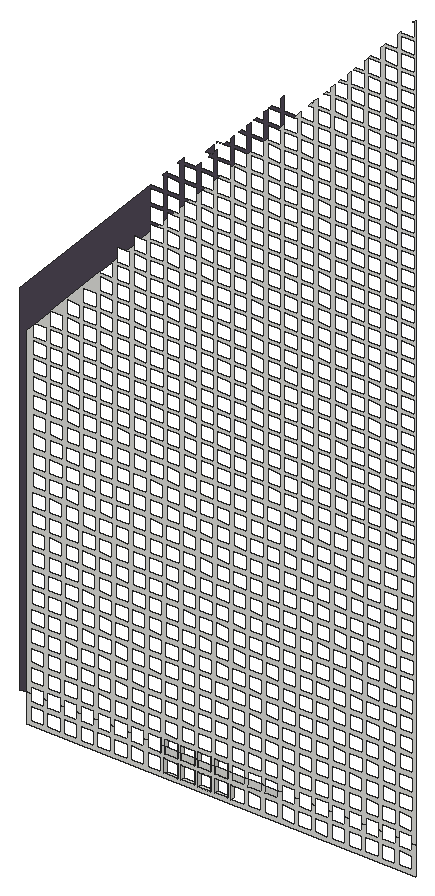
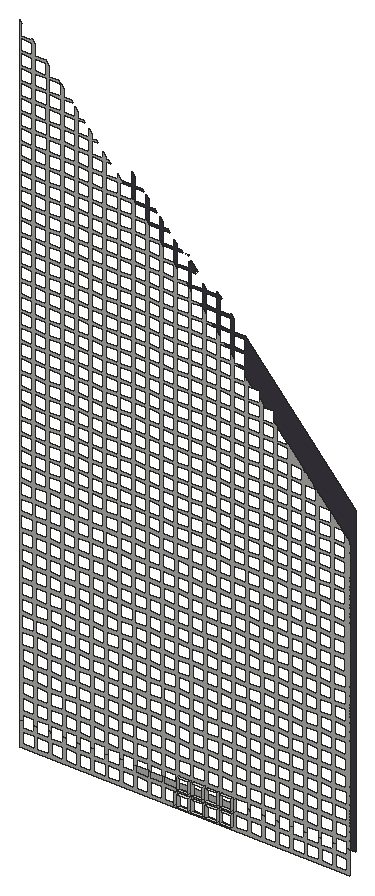
# SketchUp Ruby script. Lengths in inches.
U = 1.inch
M = Sketchup.active_model
def pt(a) = Geom::Point3d.new(a.map { |v| v * U })
def face(e, loops, mat)
  f = e.add_face(loops[0].map { |a| pt(a) })
  loops[1..].each { |l| e.add_face(l.map { |a| pt(a) }).erase! }
  f.material = f.back_material = mat if mat
  f
end
# faces: each face lists its corners as indices into pts; further lists are holes
def faces(e, pts, list, mat = nil) = list.each { |f| face(e, (f[0].is_a?(Array) ? f : [f]).map { |l| l.map { |i| pts[i] } }, mat) }
# xy, xz, yz: faces in a plane at the given z, y or x. An outline is a flat list of corners, or four numbers for a rectangle; further outlines are holes
def ring(l) = l.size == 4 ? [[l[0], l[1]], [l[2], l[1]], [l[2], l[3]], [l[0], l[3]]] : l.each_slice(2).to_a
def flat(e, list, mat, &to3) = list.each { |f| face(e, (f[0].is_a?(Array) ? f : [f]).map { |l| ring(l).map { |u, v| to3.(u, v) } }, mat) }
def xy(e, z, list, mat = nil) = flat(e, list, mat) { |x, y| [x, y, z] }
def xz(e, y, list, mat = nil) = flat(e, list, mat) { |x, z| [x, y, z] }
def yz(e, x, list, mat = nil) = flat(e, list, mat) { |y, z| [x, y, z] }
def lines(e, pts, list) = list.each { |a, b| e.add_line(pt(pts[a]), pt(pts[b])) }
# prism: a flat outline (further loops are holes) pulled along v
def prism(e, loops, v, mat = nil)
  f = face(e, loops, mat); d = Geom::Vector3d.new(v.map { |x| x * U })
  f.pushpull(f.normal.samedirection?(d) ? d.length : -d.length)
end
def box(e, o, s, mat = nil) = prism(e, [[o, [o[0] + s[0], o[1], o[2]], [o[0] + s[0], o[1] + s[1], o[2]], [o[0], o[1] + s[1], o[2]]]], [0, 0, s[2]], mat)
def at(x, y, z, deg = 0) = Geom::Transformation.translation(pt([x, y, z])) * Geom::Transformation.rotation(ORIGIN, Z_AXIS, deg.degrees)
def axes(o, x, y, z) = Geom::Transformation.new([*x, 0, *y, 0, *z, 0, *pt(o).to_a, 1])
def part(name) = M.definitions.add(name)
# library, detail: a bought-in or finely detailed component or shape, given as its bounding box
def library(name, o, s) = part(name).tap { |d| box(d.entities, o, s) }
def detail(e, o, s) = box(e.add_group.entities, o, s)
def put(e, d, t, mat = nil) = e.add_instance(d, t).tap { |i| i.material = mat if mat }
def group(e, t, mat = nil) = e.add_group.tap { |g| g.transformation = t; g.material = mat if mat }.entities
root = M.entities
M.materials.add("[Color M06]").color = [79, 71, 84]
xy(root,259.68,[[974.76,2332.13,977.07,2332.76],[977.67,2332.13,979.99,2332.76],[980.59,2332.13,982.9,2332.76],[983.5,2332.13,985.8125,2332.76]])
xy(root,262,[[974.76,2332.13,977.07,2332.76],[977.67,2332.13,979.99,2332.76],[980.59,2332.13,982.9,2332.76],[983.5,2332.13,985.8125,2332.76]])
xy(root,262.73,[[974.79,2332.13,977.1,2332.76],[977.7,2332.13,980.02,2332.76],[980.62,2332.13,982.93,2332.76],[983.53,2332.13,985.84,2332.76]])
xy(root,265.04,[[974.79,2332.13,977.1,2332.76],[977.7,2332.13,980.02,2332.76],[980.62,2332.13,982.93,2332.76],[983.53,2332.13,985.84,2332.76]])
xz(root,2332.13,[[[950.85,258.95,1018.44,258.95,1018.44,263.89,1017.87,263.89,1017.87,262.73,1015.56,262.73,1015.56,263.89,1014.96,263.89,1014.96,262.73,1012.65,262.73,1012.65,263.89,1012.05,263.89,1012.05,262.73,1009.74,262.73,1009.74,263.89,1009.14,263.89,1009.14,262.73,1006.82,262.73,1006.82,263.89,1006.22,263.89,1006.22,262.73,1003.91,262.73,1003.91,263.89,1003.3125,263.89,1003.3125,262.73,1001,262.73,1001,263.89,1000.4,263.89,1000.4,262.73,998.09,262.73,998.09,263.89,997.49,263.89,997.49,262.73,995.18,262.73,995.18,263.89,994.58,263.89,994.58,262.73,992.26,262.73,992.26,263.89,991.66,263.89,991.66,262.73,989.35,262.73,989.35,263.89,988.75,263.89,988.75,262.73,986.4375,262.73,986.4375,263.89,985.84,263.89,985.84,262.73,983.53,262.73,983.53,263.89,982.93,263.89,982.93,262.73,980.62,262.73,980.62,263.89,980.02,263.89,980.02,262.73,977.7,262.73,977.7,263.89,977.1,263.89,977.1,262.73,974.79,262.73,974.79,263.89,974.19,263.89,974.19,262.73,971.88,262.73,971.88,263.89,971.28,263.89,971.28,262.73,968.97,262.73,968.97,263.89,968.37,263.89,968.37,262.73,966.06,262.73,966.06,263.89,965.46,263.89,965.46,262.73,963.14,262.73,963.14,263.89,962.54,263.89,962.54,262.73,960.23,262.73,960.23,263.89,959.63,263.89,959.63,262.73,957.32,262.73,957.32,263.89,956.72,263.89,956.72,262.73,954.41,262.73,954.41,263.89,953.81,263.89,953.81,262.73,951.49,262.73,951.49,263.89,950.85,263.89],[1015.53,259.68,1017.84,262],[1012.62,259.68,1014.93,262],[1009.71,259.68,1012.02,262],[1006.79,259.68,1009.11,262],[1003.88,259.68,1006.2,262],[1000.97,259.68,1003.28,262],[998.06,259.68,1000.37,262],[995.15,259.68,997.46,262],[992.23,259.68,994.55,262],[989.32,259.68,991.63,262],[986.41,259.68,988.72,262],[983.5,259.68,985.8125,262],[980.59,259.68,982.9,262],[977.67,259.68,979.99,262],[974.76,259.68,977.07,262],[971.85,259.68,974.16,262],[968.9375,259.68,971.25,262],[966.03,259.68,968.34,262],[963.11,259.68,965.43,262],[960.2,259.68,962.51,262],[957.29,259.68,959.6,262],[954.38,259.68,956.69,262],[951.47,259.68,953.78,262]],[974.79,262.73,977.1,263.89],[977.7,262.73,980.02,263.89],[980.62,262.73,982.93,263.89],[983.53,262.73,985.84,263.89],
  [986.4375,262.73,988.75,263.89],[989.35,262.73,991.66,263.89],[992.26,262.73,994.58,263.89],[[950.85,263.89,951.49,263.89,951.49,265.04,953.81,265.04,953.81,263.89,954.41,263.89,954.41,265.04,956.72,265.04,956.72,263.89,957.32,263.89,957.32,265.04,959.63,265.04,959.63,263.89,960.23,263.89,960.23,265.04,962.54,265.04,962.54,263.89,963.14,263.89,963.14,265.04,965.46,265.04,965.46,263.89,966.06,263.89,966.06,265.04,968.37,265.04,968.37,263.89,968.97,263.89,968.97,265.04,971.28,265.04,971.28,263.89,971.88,263.89,971.88,265.04,974.19,265.04,974.19,263.89,974.79,263.89,974.79,265.04,977.1,265.04,977.1,263.89,977.7,263.89,977.7,265.04,980.02,265.04,980.02,263.89,980.62,263.89,980.62,265.04,982.93,265.04,982.93,263.89,983.53,263.89,983.53,265.04,985.84,265.04,985.84,263.89,986.4375,263.89,986.4375,265.04,988.75,265.04,988.75,263.89,989.35,263.89,989.35,265.04,991.66,265.04,991.66,263.89,992.26,263.89,992.26,265.04,994.58,265.04,994.58,263.89,995.18,263.89,995.18,265.04,997.49,265.04,997.49,263.89,998.09,263.89,998.09,265.04,1000.4,265.04,1000.4,263.89,1001,263.89,1001,265.04,1003.3125,265.04,1003.3125,263.89,1003.91,263.89,1003.91,265.04,1006.22,265.04,1006.22,263.89,1006.82,263.89,1006.82,265.04,1009.14,265.04,1009.14,263.89,1009.74,263.89,1009.74,265.04,1012.05,265.04,1012.05,263.89,1012.65,263.89,1012.65,265.04,1014.96,265.04,1014.96,263.89,1015.56,263.89,1015.56,265.04,1017.87,265.04,1017.87,263.89,1018.44,263.89,1018.44,392.36,1018.01,391.9,1018.31,391.9,1018.31,389.59,1015.99,389.59,1015.99,389.75,1015.4,389.11,1015.4,386.84,1013.27,386.84,1012.48,386,1012.48,384.09,1010.69,384.09,1010.37,383.75,1010.28,383.65,1012.48,383.65,1012.48,381.34,1010.17,381.34,1010.17,383.53,1009.57,382.89,1009.57,381.34,1008.11,381.34,1007.7,380.9,1009.57,380.9,1009.57,378.59,1007.26,378.59,1007.26,380.43,1006.66,379.79,1006.66,378.59,1005.53,378.59,1005.125,378.15,1006.66,378.15,1006.66,375.84,1004.35,375.84,1004.35,377.32,1003.75,376.68,1003.75,375.84,1002.96,375.84,1002.55,375.4,1003.75,375.4,1003.75,373.09,1001.43,373.09,1001.43,374.21,1000.83,373.57,1000.83,373.09,1000.38,373.09,999.91,372.59,1000.83,372.59,1000.83,370.27,998.52,370.27,998.52,371.11,997.92,370.47,997.92,370.27,997.74,370.27,997.27,369.77,997.92,369.77,997.92,367.46,995.61,367.46,995.61,368,994.64,366.96,995.01,366.96,995.01,364.65,992.7,364.65,992.7,364.89,992,364.15,992.1,364.15,992.1,361.84,989.84,361.84,989.1875,361.14,989.1875,359.02,987.2,359.02,986.27,358.04,986.27,356.21,984.5625,356.21,984.09,355.71,986.27,355.71,986.27,353.4,983.96,353.4,983.96,355.57,983.36,354.93,983.36,353.4,981.93,353.4,981.46,352.9,983.36,352.9,983.36,350.59,981.05,350.59,981.05,352.46,980.45,351.82,980.45,350.59,979.29,350.59,978.82,350.09,980.45,350.09,980.45,347.77,978.14,347.77,978.14,349.36,977.54,348.72,977.54,347.77,976.65,347.77,976.1875,347.27,977.54,347.27,977.54,344.96,975.23,344.96,975.23,346.25,974.625,345.61,974.625,344.96,974.02,344.96,973.55,344.46,974.625,344.46,974.625,342.15,972.3125,342.15,972.3125,343.14,970.91,341.65,971.71,341.65,971.71,339.34,969.4,339.34,969.4,340.04,968.28,338.84,968.8,338.84,968.8,336.52,966.49,336.52,966.49,336.93,965.64,336.02,965.89,336.02,965.89,333.71,963.58,333.71,963.58,333.82,955.1,324.77,957.15,324.77,957.15,322.46,954.84,322.46,954.84,324.5,952.46,321.96,954.24,321.96,954.24,319.65,951.93,319.65,951.93,321.39,950.85,320.24],[1015.99,375.84,1018.31,378.15],[1013.06,373.09,1015.37,375.4],[1015.99,373.09,1018.31,375.4],[1013.06,370.27,1015.37,372.59],[1015.99,370.27,1018.31,372.59],[1004.32,370.27,1006.63,372.59],[1007.26,370.27,1009.57,372.59],[1007.23,373.09,1009.55,375.4],[1010.17,373.09,1012.48,375.4],[1010.15,375.84,1012.46,378.15],[1013.08,375.84,1015.4,378.15],[1013.06,378.59,1015.37,380.9],[1015.99,378.59,1018.31,380.9],[1013.06,381.34,1015.37,383.65],[1015.99,381.34,1018.31,383.65],[983.96,350.59,986.27,352.9],[981.05,347.77,983.36,350.09],[983.96,347.77,986.27,350.09],[978.14,344.96,980.45,347.27],[981.05,344.96,983.36,347.27],[983.96,344.96,986.27,347.27],[986.875,344.96,989.1875,347.27],[989.79,344.96,992.1,347.27],[992.7,344.96,995.01,347.27],[995.61,344.96,997.92,347.27],[998.52,344.96,1000.83,347.27],[1001.43,344.96,1003.75,347.27],[1004.35,344.96,1006.66,347.27],[1007.26,344.96,1009.57,347.27],[1010.17,344.96,1012.48,347.27],[1013.08,344.96,1015.4,347.27],[1015.99,344.96,1018.31,347.27],[986.875,347.77,989.1875,350.09],[989.79,347.77,992.1,350.09],[992.7,347.77,995.01,350.09],[995.61,347.77,997.92,350.09],[998.52,347.77,1000.83,350.09],[1001.43,347.77,1003.75,350.09],[1004.35,347.77,1006.66,350.09],[1007.26,347.77,1009.57,350.09],[1010.17,347.77,1012.48,350.09],[1013.08,347.77,1015.4,350.09],[1015.99,347.77,1018.31,350.09],[986.875,350.59,989.1875,352.9],[989.79,350.59,992.1,352.9],[992.7,350.59,995.01,352.9],[995.61,350.59,997.92,352.9],[998.52,350.59,1000.83,352.9],[1001.43,350.59,1003.75,352.9],[1004.35,350.59,1006.66,352.9],[1007.26,350.59,1009.57,352.9],[1010.17,350.59,1012.48,352.9],[1013.08,350.59,1015.4,352.9],[1015.99,350.59,1018.31,352.9],[986.875,353.4,989.1875,355.71],[989.79,353.4,992.1,355.71],[992.7,353.4,995.01,355.71],[995.61,353.4,997.92,355.71],[998.52,353.4,1000.83,355.71],[1001.43,353.4,1003.75,355.71],[1004.35,353.4,1006.66,355.71],[1007.26,353.4,1009.57,355.71],[1010.17,353.4,1012.48,355.71],[1013.08,353.4,1015.4,355.71],[1015.99,353.4,1018.31,355.71],[998.52,367.46,1000.83,369.77],[1001.43,367.46,1003.75,369.77],[1010.17,367.46,1012.48,369.77],[1015.99,367.46,1018.31,369.77],[1007.26,367.46,1009.57,369.77],[1004.35,367.46,1006.66,369.77],[1013.08,367.46,1015.4,369.77],[998.52,364.65,1000.83,366.96],[1004.35,364.65,1006.66,366.96],[1013.08,364.65,1015.4,366.96],[1010.17,364.65,1012.48,366.96],[1001.43,364.65,1003.75,366.96],[1007.26,364.65,1009.57,366.96],[1015.99,364.65,1018.31,366.96],[995.61,364.65,997.92,366.96],[1007.26,361.84,1009.57,364.15],[1013.08,361.84,1015.4,364.15],[1001.43,361.84,1003.75,364.15],[1004.35,361.84,1006.66,364.15],[1015.99,361.84,1018.31,364.15],[995.61,361.84,997.92,364.15],[992.7,361.84,995.01,364.15],[998.52,361.84,1000.83,364.15],[1010.17,361.84,1012.48,364.15],[1007.26,359.02,1009.57,361.34],[1013.08,359.02,1015.4,361.34],[1001.43,359.02,1003.75,361.34],[989.79,359.02,992.1,361.34],[1015.99,359.02,1018.31,361.34],[1004.35,359.02,1006.66,361.34],[995.61,359.02,997.92,361.34],[992.7,359.02,995.01,361.34],[1010.17,359.02,1012.48,361.34],[998.52,359.02,1000.83,361.34],[1010.17,356.21,1012.48,358.52],[998.52,356.21,1000.83,358.52],[992.7,356.21,995.01,358.52],[1004.35,356.21,1006.66,358.52],[1015.99,356.21,1018.31,358.52],[986.875,356.21,989.1875,358.52],[995.61,356.21,997.92,358.52],[989.79,356.21,992.1,358.52],[1001.43,356.21,1003.75,358.52],[1013.08,356.21,1015.4,358.52],[1007.26,356.21,1009.57,358.52],[975.23,342.15,977.54,344.46],[978.14,342.15,980.45,344.46],[981.05,342.15,983.36,344.46],[983.96,342.15,986.27,344.46],[986.875,342.15,989.1875,344.46],[989.79,342.15,992.1,344.46],[992.7,342.15,995.01,344.46],[995.61,342.15,997.92,344.46],[998.52,342.15,1000.83,344.46],[1001.43,342.15,1003.75,344.46],[1004.35,342.15,1006.66,344.46],[1007.26,342.15,1009.57,344.46],[1010.17,342.15,1012.48,344.46],[1013.08,342.15,1015.4,344.46],[1015.99,342.15,1018.31,344.46],[972.3125,339.34,974.625,341.65],[975.23,339.34,977.54,341.65],[978.14,339.34,980.45,341.65],[981.05,339.34,983.36,341.65],[983.96,339.34,986.27,341.65],[986.875,339.34,989.1875,341.65],[989.79,339.34,992.1,341.65],[992.7,339.34,995.01,341.65],[995.61,339.34,997.92,341.65],[998.52,339.34,1000.83,341.65],[1001.43,339.34,1003.75,341.65],[1004.35,339.34,1006.66,341.65],[1007.26,339.34,1009.57,341.65],[1010.17,339.34,1012.48,341.65],[1013.08,339.34,1015.4,341.65],[1015.99,339.34,1018.31,341.65],[969.4,336.52,971.71,338.84],[972.3125,336.52,974.625,338.84],[975.23,336.52,977.54,338.84],[978.14,336.52,980.45,338.84],[981.05,336.52,983.36,338.84],[983.96,336.52,986.27,338.84],[986.875,336.52,989.1875,338.84],[989.79,336.52,992.1,338.84],[992.7,336.52,995.01,338.84],[995.61,336.52,997.92,338.84],[998.52,336.52,1000.83,338.84],[1001.43,336.52,1003.75,338.84],[1004.35,336.52,1006.66,338.84],[1007.26,336.52,1009.57,338.84],[1010.17,336.52,1012.48,338.84],[1013.08,336.52,1015.4,338.84],[1015.99,336.52,1018.31,338.84],[966.49,333.71,968.8,336.02],[969.4,333.71,971.71,336.02],[972.3125,333.71,974.625,336.02],[975.23,333.71,977.54,336.02],[978.14,333.71,980.45,336.02],[981.05,333.71,983.36,336.02],[983.96,333.71,986.27,336.02],[986.875,333.71,989.1875,336.02],[989.79,333.71,992.1,336.02],[992.7,333.71,995.01,336.02],[995.61,333.71,997.92,336.02],[998.52,333.71,1000.83,336.02],[1001.43,333.71,1003.75,336.02],[1004.35,333.71,1006.66,336.02],[1007.26,333.71,1009.57,336.02],[1010.17,333.71,1012.48,336.02],[1013.08,333.71,1015.4,336.02],[1015.99,333.71,1018.31,336.02],[963.58,330.9,965.89,333.21],[966.49,330.9,968.8,333.21],[969.4,330.9,971.71,333.21],[972.3125,330.9,974.625,333.21],[975.23,330.9,977.54,333.21],[978.14,330.9,980.45,333.21],[981.05,330.9,983.36,333.21],[983.96,330.9,986.27,333.21],[986.875,330.9,989.1875,333.21],[989.79,330.9,992.1,333.21],[992.7,330.9,995.01,333.21],[995.61,330.9,997.92,333.21],[998.52,330.9,1000.83,333.21],[1001.43,330.9,1003.75,333.21],[1004.35,330.9,1006.66,333.21],[1007.26,330.9,1009.57,333.21],[1010.17,330.9,1012.48,333.21],[1013.08,330.9,1015.4,333.21],[1015.99,330.9,1018.31,333.21],[960.67,328.09,962.98,330.4],[963.58,328.09,965.89,330.4],[966.49,328.09,968.8,330.4],[969.4,328.09,971.71,330.4],[972.3125,328.09,974.625,330.4],[975.23,328.09,977.54,330.4],[978.14,328.09,980.45,330.4],[981.05,328.09,983.36,330.4],[983.96,328.09,986.27,330.4],[986.875,328.09,989.1875,330.4],[989.79,328.09,992.1,330.4],[992.7,328.09,995.01,330.4],[995.61,328.09,997.92,330.4],[998.52,328.09,1000.83,330.4],[1001.43,328.09,1003.75,330.4],[1004.35,328.09,1006.66,330.4],[1007.26,328.09,1009.57,330.4],[1010.17,328.09,1012.48,330.4],[1013.08,328.09,1015.4,330.4],[1015.99,328.09,1018.31,330.4],[957.75,325.27,960.07,327.59],[960.67,325.27,962.98,327.59],[963.58,325.27,965.89,327.59],[966.49,325.27,968.8,327.59],[969.4,325.27,971.71,327.59],[972.3125,325.27,974.625,327.59],[975.23,325.27,977.54,327.59],[978.14,325.27,980.45,327.59],[981.05,325.27,983.36,327.59],[983.96,325.27,986.27,327.59],[986.875,325.27,989.1875,327.59],[989.79,325.27,992.1,327.59],[992.7,325.27,995.01,327.59],[995.61,325.27,997.92,327.59],[998.52,325.27,1000.83,327.59],[1001.43,325.27,1003.75,327.59],[1004.35,325.27,1006.66,327.59],[1007.26,325.27,1009.57,327.59],[1010.17,325.27,1012.48,327.59],[1013.08,325.27,1015.4,327.59],[1015.99,325.27,1018.31,327.59],[957.75,322.46,960.07,324.77],[960.67,322.46,962.98,324.77],[963.58,322.46,965.89,324.77],[966.49,322.46,968.8,324.77],[969.4,322.46,971.71,324.77],[972.3125,322.46,974.625,324.77],[975.23,322.46,977.54,324.77],[978.14,322.46,980.45,324.77],[981.05,322.46,983.36,324.77],[983.96,322.46,986.27,324.77],[986.875,322.46,989.1875,324.77],[989.79,322.46,992.1,324.77],[992.7,322.46,995.01,324.77],[995.61,322.46,997.92,324.77],[998.52,322.46,1000.83,324.77],[1001.43,322.46,1003.75,324.77],[1004.35,322.46,1006.66,324.77],[1007.26,322.46,1009.57,324.77],[1010.17,322.46,1012.48,324.77],[1013.08,322.46,1015.4,324.77],[1015.99,322.46,1018.31,324.77],[954.84,319.65,957.15,321.96],[957.75,319.65,960.07,321.96],[960.67,319.65,962.98,321.96],[963.58,319.65,965.89,321.96],[966.49,319.65,968.8,321.96],[969.4,319.65,971.71,321.96],[972.3125,319.65,974.625,321.96],[975.23,319.65,977.54,321.96],[978.14,319.65,980.45,321.96],[981.05,319.65,983.36,321.96],[983.96,319.65,986.27,321.96],[986.875,319.65,989.1875,321.96],[989.79,319.65,992.1,321.96],[992.7,319.65,995.01,321.96],[995.61,319.65,997.92,321.96],[998.52,319.65,1000.83,321.96],[1001.43,319.65,1003.75,321.96],[1004.35,319.65,1006.66,321.96],[1007.26,319.65,1009.57,321.96],[1010.17,319.65,1012.48,321.96],[1013.08,319.65,1015.4,321.96],[1015.99,319.65,1018.31,321.96],[951.93,316.84,954.24,319.15],[954.84,316.84,957.15,319.15],[957.75,316.84,960.07,319.15],[960.67,316.84,962.98,319.15],[963.58,316.84,965.89,319.15],[966.49,316.84,968.8,319.15],[969.4,316.84,971.71,319.15],[972.3125,316.84,974.625,319.15],[975.23,316.84,977.54,319.15],[978.14,316.84,980.45,319.15],[981.05,316.84,983.36,319.15],[983.96,316.84,986.27,319.15],[986.875,316.84,989.1875,319.15],[989.79,316.84,992.1,319.15],[992.7,316.84,995.01,319.15],[995.61,316.84,997.92,319.15],[998.52,316.84,1000.83,319.15],[1001.43,316.84,1003.75,319.15],[1004.35,316.84,1006.66,319.15],[1007.26,316.84,1009.57,319.15],[1010.17,316.84,1012.48,319.15],[1013.08,316.84,1015.4,319.15],[1015.99,316.84,1018.31,319.15],[951.93,314.02,954.24,316.34],[954.84,314.02,957.15,316.34],[957.75,314.02,960.07,316.34],[960.67,314.02,962.98,316.34],[963.58,314.02,965.89,316.34],[966.49,314.02,968.8,316.34],[969.4,314.02,971.71,316.34],[972.3125,314.02,974.625,316.34],[975.23,314.02,977.54,316.34],[978.14,314.02,980.45,316.34],[981.05,314.02,983.36,316.34],[983.96,314.02,986.27,316.34],[986.875,314.02,989.1875,316.34],[989.79,314.02,992.1,316.34],[992.7,314.02,995.01,316.34],[995.61,314.02,997.92,316.34],[998.52,314.02,1000.83,316.34],[1001.43,314.02,1003.75,316.34],[1004.35,314.02,1006.66,316.34],[1007.26,314.02,1009.57,316.34],[1010.17,314.02,1012.48,316.34],[1013.08,314.02,1015.4,316.34],[1015.99,314.02,1018.31,316.34],[969.4,311.21,971.71,313.52],[972.3125,311.21,974.625,313.52],[957.75,311.21,960.07,313.52],[951.93,311.21,954.24,313.52],[1013.08,311.21,1015.4,313.52],[995.61,311.21,997.92,313.52],[983.96,311.21,986.27,313.52],[960.67,311.21,962.98,313.52],[989.79,311.21,992.1,313.52],[986.875,311.21,989.1875,313.52],[963.58,311.21,965.89,313.52],[1001.43,311.21,1003.75,313.52],[975.23,311.21,977.54,313.52],[1010.17,311.21,1012.48,313.52],[1004.35,311.21,1006.66,313.52],[954.84,311.21,957.15,313.52],[998.52,311.21,1000.83,313.52],[1007.26,311.21,1009.57,313.52],[981.05,311.21,983.36,313.52],[1015.99,311.21,1018.31,313.52],[966.49,311.21,968.8,313.52],[978.14,311.21,980.45,313.52],[992.7,311.21,995.01,313.52],[951.93,308.4,954.24,310.71],[954.84,308.4,957.15,310.71],[957.75,308.4,960.07,310.71],[960.67,308.4,962.98,310.71],[963.58,308.4,965.89,310.71],[966.49,308.4,968.8,310.71],[969.4,308.4,971.71,310.71],[972.3125,308.4,974.625,310.71],[975.23,308.4,977.54,310.71],[978.14,308.4,980.45,310.71],[981.05,308.4,983.36,310.71],[983.96,308.4,986.27,310.71],[986.875,308.4,989.1875,310.71],[989.79,308.4,992.1,310.71],[992.7,308.4,995.01,310.71],[995.61,308.4,997.92,310.71],[998.52,308.4,1000.83,310.71],[1001.43,308.4,1003.75,310.71],[1004.35,308.4,1006.66,310.71],[1007.26,308.4,1009.57,310.71],[1010.17,308.4,1012.48,310.71],[1013.08,308.4,1015.4,310.71],[1015.99,308.4,1018.31,310.71],[951.9,305.35,954.21,307.67],[954.8125,305.35,957.125,307.67],[957.72,305.35,960.04,307.67],[960.64,305.35,962.95,307.67],[963.55,305.35,965.86,307.67],[966.46,305.35,968.77,307.67],[969.375,305.35,971.6875,307.67],[972.29,305.35,974.6,307.67],[975.2,305.35,977.51,307.67],[978.11,305.35,980.42,307.67],[981.02,305.35,983.33,307.67],[983.93,305.35,986.25,307.67],[986.85,305.35,989.16,307.67],[989.76,305.35,992.07,307.67],[992.67,305.35,994.98,307.67],[995.58,305.35,997.89,307.67],[998.49,305.35,1000.81,307.67],[1001.41,305.35,1003.72,307.67],[1004.32,305.35,1006.63,307.67],[1007.23,305.35,1009.54,307.67],[1010.14,305.35,1012.45,307.67],[1013.05,305.35,1015.37,307.67],[1015.97,305.35,1018.28,307.67],[951.87,302.31,954.18,304.62],[954.78,302.31,957.1,304.62],[957.7,302.31,960.01,304.62],[960.61,302.31,962.92,304.62],[963.52,302.31,965.83,304.62],[966.43,302.31,968.74,304.62],[969.34,302.31,971.66,304.62],[972.26,302.31,974.57,304.62],[975.17,302.31,977.48,304.62],[978.08,302.31,980.39,304.62],[980.99,302.31,983.3,304.62],[983.9,302.31,986.22,304.62],[986.82,302.31,989.13,304.62],[989.73,302.31,992.04,304.62],[992.64,302.31,994.95,304.62],[995.55,302.31,997.86,304.62],[998.46,302.31,1000.78,304.62],[1001.375,302.31,1003.6875,304.62],[1004.29,302.31,1006.6,304.62],[1007.2,302.31,1009.51,304.62],[1010.11,302.31,1012.43,304.62],[1013.02,302.31,1015.34,304.62],[1015.9375,302.31,1018.25,304.62],[951.84,299.27,954.16,301.58],[954.75,299.27,957.07,301.58],[957.67,299.27,959.98,301.58],[960.58,299.27,962.89,301.58],[963.49,299.27,965.8,301.58],[966.4,299.27,968.72,301.58],[969.32,299.27,971.63,301.58],[972.23,299.27,974.54,301.58],[975.14,299.27,977.45,301.58],[978.05,299.27,980.36,301.58],[980.96,299.27,983.28,301.58],[983.875,299.27,986.1875,301.58],[986.79,299.27,989.1,301.58],[989.7,299.27,992.01,301.58],[992.61,299.27,994.92,301.58],[995.52,299.27,997.84,301.58],[998.44,299.27,1000.75,301.58],[1001.35,299.27,1003.66,301.58],[1004.26,299.27,1006.57,301.58],[1007.17,299.27,1009.48,301.58],[1010.08,299.27,1012.4,301.58],[1013,299.27,1015.31,301.58],[1015.91,299.27,1018.22,301.58],[951.8125,296.22,954.125,298.53],[954.73,296.22,957.04,298.53],[957.64,296.22,959.95,298.53],[960.55,296.22,962.86,298.53],[963.46,296.22,965.77,298.53],[966.375,296.22,968.6875,298.53],[969.29,296.22,971.6,298.53],[972.2,296.22,974.51,298.53],[975.11,296.22,977.42,298.53],[978.02,296.22,980.33,298.53],[980.93,296.22,983.25,298.53],[983.85,296.22,986.16,298.53],[986.76,296.22,989.07,298.53],[989.67,296.22,991.98,298.53],[992.58,296.22,994.89,298.53],[995.49,296.22,997.81,298.53],[998.41,296.22,1000.72,298.53],[1001.32,296.22,1003.63,298.53],[1004.23,296.22,1006.54,298.53],[1007.14,296.22,1009.46,298.53],[1010.05,296.22,1012.37,298.53],[1012.97,296.22,1015.28,298.53],[1015.88,296.22,1018.19,298.53],[951.78,293.18,954.1,295.49],[954.7,293.18,957.01,295.49],[957.61,293.18,959.92,295.49],[960.52,293.18,962.83,295.49],[963.43,293.18,965.75,295.49],[966.35,293.18,968.66,295.49],[969.26,293.18,971.57,295.49],[972.17,293.18,974.48,295.49],[975.08,293.18,977.39,295.49],[977.99,293.18,980.31,295.49],[980.91,293.18,983.22,295.49],[983.82,293.18,986.13,295.49],[986.73,293.18,989.04,295.49],[989.64,293.18,991.95,295.49],[992.55,293.18,994.87,295.49],[995.47,293.18,997.78,295.49],[998.38,293.18,1000.69,295.49],[1001.29,293.18,1003.6,295.49],[1004.2,293.18,1006.51,295.49],[1007.11,293.18,1009.43,295.49],[1010.03,293.18,1012.34,295.49],[1012.9375,293.18,1015.25,295.49],[1015.85,293.18,1018.16,295.49],[951.76,290.13,954.07,292.44],[954.67,290.13,956.98,292.44],[957.58,290.13,959.89,292.44],[960.49,290.13,962.8,292.44],[963.4,290.13,965.72,292.44],[966.32,290.13,968.63,292.44],[969.23,290.13,971.54,292.44],[972.14,290.13,974.45,292.44],[975.05,290.13,977.36,292.44],[977.96,290.13,980.28,292.44],[980.875,290.13,983.1875,292.44],[983.79,290.13,986.1,292.44],[986.7,290.13,989.01,292.44],[989.61,290.13,991.92,292.44],[992.52,290.13,994.84,292.44],[995.4375,290.13,997.75,292.44],[998.35,290.13,1000.66,292.44],[1001.26,290.13,1003.57,292.44],[1004.17,290.13,1006.49,292.44],[1007.08,290.13,1009.4,292.44],[1010,290.13,1012.31,292.44],[1012.91,290.13,1015.22,292.44],[1015.82,290.13,1018.13,292.44],[951.73,287.09,954.04,289.4],[954.64,287.09,956.95,289.4],[957.55,287.09,959.86,289.4],[960.46,287.09,962.78,289.4],[963.375,287.09,965.6875,289.4],[966.29,287.09,968.6,289.4],[969.2,287.09,971.51,289.4],[972.11,287.09,974.42,289.4],[975.02,287.09,977.34,289.4],[977.94,287.09,980.25,289.4],[980.85,287.09,983.16,289.4],[983.76,287.09,986.07,289.4],[986.67,287.09,988.98,289.4],[989.58,287.09,991.9,289.4],[992.5,287.09,994.81,289.4],[995.41,287.09,997.72,289.4],[998.32,287.09,1000.63,289.4],[1001.23,287.09,1003.54,289.4],[1004.14,287.09,1006.46,289.4],[1007.06,287.09,1009.37,289.4],[1009.97,287.09,1012.28,289.4],[1012.88,287.09,1015.19,289.4],[1015.79,287.09,1018.1,289.4],[951.7,284.04,954.01,286.35],[954.61,284.04,956.92,286.35],[957.52,284.04,959.83,286.35],[960.43,284.04,962.75,286.35],[963.35,284.04,965.66,286.35],[966.26,284.04,968.57,286.35],[969.17,284.04,971.48,286.35],[972.08,284.04,974.39,286.35],[974.99,284.04,977.31,286.35],[977.91,284.04,980.22,286.35],[980.82,284.04,983.13,286.35],[983.73,284.04,986.04,286.35],[986.64,284.04,988.95,286.35],[989.55,284.04,991.87,286.35],[992.47,284.04,994.78,286.35],[995.38,284.04,997.69,286.35],[998.29,284.04,1000.6,286.35],[1001.2,284.04,1003.52,286.35],[1004.11,284.04,1006.43,286.35],[1007.03,284.04,1009.34,286.35],[1009.9375,284.04,1012.25,286.35],[1012.85,284.04,1015.16,286.35],[1015.76,284.04,1018.08,286.35],[951.67,281,953.98,283.31],[954.58,281,956.89,283.31],[957.49,281,959.81,283.31],[960.41,281,962.72,283.31],[963.32,281,965.63,283.31],[966.23,281,968.54,283.31],[969.14,281,971.45,283.31],[972.05,281,974.37,283.31],[974.97,281,977.28,283.31],[977.88,281,980.19,283.31],[980.79,281,983.1,283.31],[983.7,281,986.01,283.31],[986.61,281,988.93,283.31],[989.53,281,991.84,283.31],[992.4375,281,994.75,283.31],[995.35,281,997.66,283.31],[998.26,281,1000.57,283.31],[1001.17,281,1003.49,283.31],[1004.09,281,1006.4,283.31],[1007,281,1009.31,283.31],[1009.91,281,1012.22,283.31],[1012.82,281,1015.13,283.31],[1015.73,281,1018.05,283.31],[951.64,277.95,953.95,280.26],[954.55,277.95,956.86,280.26],[957.46,277.95,959.78,280.26],[960.375,277.95,962.6875,280.26],[963.29,277.95,965.6,280.26],[966.2,277.95,968.51,280.26],[969.11,277.95,971.42,280.26],[972.02,277.95,974.34,280.26],[974.9375,277.95,977.25,280.26],[977.85,277.95,980.16,280.26],[980.76,277.95,983.07,280.26],[983.67,277.95,985.98,280.26],[986.58,277.95,988.9,280.26],[989.5,277.95,991.81,280.26],[992.41,277.95,994.72,280.26],[995.32,277.95,997.63,280.26],[998.23,277.95,1000.55,280.26],[1001.14,277.95,1003.46,280.26],[1004.06,277.95,1006.37,280.26],[1006.97,277.95,1009.28,280.26],[1009.88,277.95,1012.19,280.26],[1012.79,277.95,1015.11,280.26],[1015.7,277.95,1018.02,280.26],[951.61,274.91,953.92,277.22],[954.52,274.91,956.84,277.22],[957.44,274.91,959.75,277.22],[960.35,274.91,962.66,277.22],[963.26,274.91,965.57,277.22],[966.17,274.91,968.48,277.22],[969.08,274.91,971.4,277.22],[972,274.91,974.31,277.22],[974.91,274.91,977.22,277.22],[977.82,274.91,980.13,277.22],[980.73,274.91,983.04,277.22],[983.64,274.91,985.96,277.22],[986.56,274.91,988.87,277.22],[989.47,274.91,991.78,277.22],[992.38,274.91,994.69,277.22],[995.29,274.91,997.6,277.22],[998.2,274.91,1000.52,277.22],[1001.12,274.91,1003.43,277.22],[1004.03,274.91,1006.34,277.22],[1006.94,274.91,1009.25,277.22],[1009.85,274.91,1012.16,277.22],[1012.76,274.91,1015.08,277.22],[1015.68,274.91,1017.99,277.22],[951.58,271.86,953.89,274.17],[954.49,271.86,956.81,274.17],[957.41,271.86,959.72,274.17],[960.32,271.86,962.63,274.17],[963.23,271.86,965.54,274.17],[966.14,271.86,968.45,274.17],[969.05,271.86,971.37,274.17],[971.97,271.86,974.28,274.17],[974.88,271.86,977.19,274.17],[977.79,271.86,980.1,274.17],[980.7,271.86,983.01,274.17],[983.61,271.86,985.93,274.17],[986.53,271.86,988.84,274.17],[989.4375,271.86,991.75,274.17],[992.35,271.86,994.66,274.17],[995.26,271.86,997.57,274.17],[998.17,271.86,1000.49,274.17],[1001.09,271.86,1003.4,274.17],[1004,271.86,1006.3125,274.17],[1006.91,271.86,1009.22,274.17],[1009.82,271.86,1012.14,274.17],[1012.73,271.86,1015.05,274.17],[1015.65,271.86,1017.96,274.17],[951.55,268.82,953.87,271.13],[954.46,268.82,956.78,271.13],[957.38,268.82,959.69,271.13],[960.29,268.82,962.6,271.13],[963.2,268.82,965.51,271.13],[966.11,268.82,968.43,271.13],[969.03,268.82,971.34,271.13],[971.9375,268.82,974.25,271.13],[974.85,268.82,977.16,271.13],[977.76,268.82,980.07,271.13],[980.67,268.82,982.99,271.13],[983.59,268.82,985.9,271.13],[986.5,268.82,988.81,271.13],[989.41,268.82,991.72,271.13],[992.32,268.82,994.63,271.13],[995.23,268.82,997.55,271.13],[998.15,268.82,1000.46,271.13],[1001.06,268.82,1003.37,271.13],[1003.97,268.82,1006.28,271.13],[1006.88,268.82,1009.19,271.13],[1009.79,268.82,1012.11,271.13],[1012.71,268.82,1015.02,271.13],[1015.62,268.82,1017.93,271.13],[951.52,265.77,953.84,268.09],[954.4375,265.77,956.75,268.09],[957.35,265.77,959.66,268.09],[960.26,265.77,962.57,268.09],[963.17,265.77,965.48,268.09],[966.08,265.77,968.4,268.09],[969,265.77,971.31,268.09],[971.91,265.77,974.22,268.09],[974.82,265.77,977.13,268.09],[977.73,265.77,980.04,268.09],[980.64,265.77,982.96,268.09],[983.56,265.77,985.87,268.09],[986.47,265.77,988.78,268.09],[989.38,265.77,991.69,268.09],[992.29,265.77,994.6,268.09],[995.2,265.77,997.52,268.09],[998.12,265.77,1000.43,268.09],[1001.03,265.77,1003.34,268.09],[1003.94,265.77,1006.25,268.09],[1006.85,265.77,1009.17,268.09],[1009.76,265.77,1012.08,268.09],[1012.68,265.77,1014.99,268.09],[1015.59,265.77,1017.9,268.09],[1015.99,384.09,1018.31,386.4],[1013.08,384.09,1015.4,386.4],[1015.99,386.84,1018.31,389.15],[1010.17,370.27,1010.17,372.47,1010.28,372.59,1012.48,372.59,1012.48,370.27],[1007.26,375.84,1007.26,378.03,1007.37,378.15,1009.57,378.15,1009.57,375.84],[1010.17,378.59,1010.17,380.78,1010.28,380.9,1012.48,380.9,1012.48,378.59],[1001.43,370.27,1001.43,372.47,1001.54,372.59,1003.75,372.59,1003.75,370.27],[1004.35,373.09,1004.35,375.28,1004.46,375.4,1006.66,375.4,1006.66,373.09]]])
xz(root,2332.13,[[[949.71,263.89,950.85,263.89,950.85,320.24,951.93,321.39,952.46,321.96,954.84,324.5,954.84,324.77,955.1,324.77,963.58,333.82,965.64,336.02,966.49,336.93,966.49,338.84,968.28,338.84,969.4,340.04,969.4,341.65,970.91,341.65,972.3125,343.14,972.3125,344.46,973.55,344.46,974.02,344.96,972.3125,344.96,972.3125,347.27,974.625,347.27,974.625,345.61,975.23,346.25,975.23,347.27,976.1875,347.27,976.65,347.77,975.23,347.77,975.23,350.09,977.54,350.09,977.54,348.72,978.14,349.36,978.14,350.09,978.82,350.09,979.29,350.59,978.14,350.59,978.14,352.9,980.45,352.9,980.45,351.82,981.05,352.46,981.05,352.9,981.46,352.9,981.93,353.4,981.05,353.4,981.05,355.71,983.36,355.71,983.36,354.93,983.96,355.57,983.96,355.71,984.09,355.71,984.5625,356.21,983.96,356.21,983.96,358.52,986.27,358.52,986.27,358.04,987.2,359.02,986.875,359.02,986.875,361.34,989.1875,361.34,989.1875,361.14,989.84,361.84,989.79,361.84,989.79,364.15,992,364.15,992.7,364.89,992.7,366.96,994.64,366.96,995.61,368,995.61,369.77,997.27,369.77,997.74,370.27,995.61,370.27,995.61,372.52,995.01,371.88,995.01,370.27,993.5,370.27,993.03,369.77,995.01,369.77,995.01,367.46,992.7,367.46,992.7,369.42,992.1,368.78,992.1,367.46,990.85,367.46,990.38,366.96,992.1,366.96,992.1,364.65,989.79,364.65,989.79,366.33,989.1875,365.69,989.1875,364.65,988.21,364.65,987.74,364.15,989.1875,364.15,989.1875,361.84,986.875,361.84,986.875,363.23,986.27,362.6,986.27,361.84,985.56,361.84,985.09,361.34,984.09,361.34,983.96,361.2,983.96,361.34,986.27,361.34,986.27,359.02,983.96,359.02,983.96,360.14,983.36,359.5,983.36,360.56,981.93,359.02,982.91,359.02,982.44,358.52,983.36,358.52,983.36,356.21,981.05,356.21,981.05,357.05,980.45,356.41,980.45,356.21,978.14,356.21,978.14,356.71,977.2,355.71,977.54,355.71,977.54,353.4,975.23,353.4,975.23,353.62,974.55,352.9,974.625,352.9,974.625,350.59,972.375,350.59,949.71,326.5],[978.14,353.4,980.45,355.71],[972.3125,347.77,974.625,350.09],[975.23,350.59,977.54,352.9],[982.91,359.02,983.36,359.5,983.36,359.02]]],"[Color M06]")
yz(root,974.19,[[2332.13,262.73,2332.76,265.04]])
yz(root,974.76,[[2332.13,259.68,2332.76,262]])
yz(root,974.79,[[2332.13,262.73,2332.76,265.04]])
yz(root,977.07,[[2332.13,259.68,2332.76,262]])
yz(root,977.1,[[2332.13,262.73,2332.76,265.04]])
yz(root,977.67,[[2332.13,259.68,2332.76,262]])
yz(root,977.7,[[2332.13,262.73,2332.76,265.04]])
yz(root,979.99,[[2332.13,259.68,2332.76,262]])
yz(root,980.02,[[2332.13,262.73,2332.76,265.04]])
yz(root,980.59,[[2332.13,259.68,2332.76,262]])
yz(root,980.62,[[2332.13,262.73,2332.76,265.04]])
yz(root,982.9,[[2332.13,259.68,2332.76,262]])
yz(root,982.93,[[2332.13,262.73,2332.76,265.04]])
yz(root,983.5,[[2332.13,259.68,2332.76,262]])
yz(root,983.53,[[2332.13,262.73,2332.76,265.04]])
yz(root,985.8125,[[2332.13,259.68,2332.76,262]])
yz(root,985.84,[[2332.13,262.73,2332.76,265.04]])
yz(root,986.41,[[2332.13,259.68,2332.76,262]])
